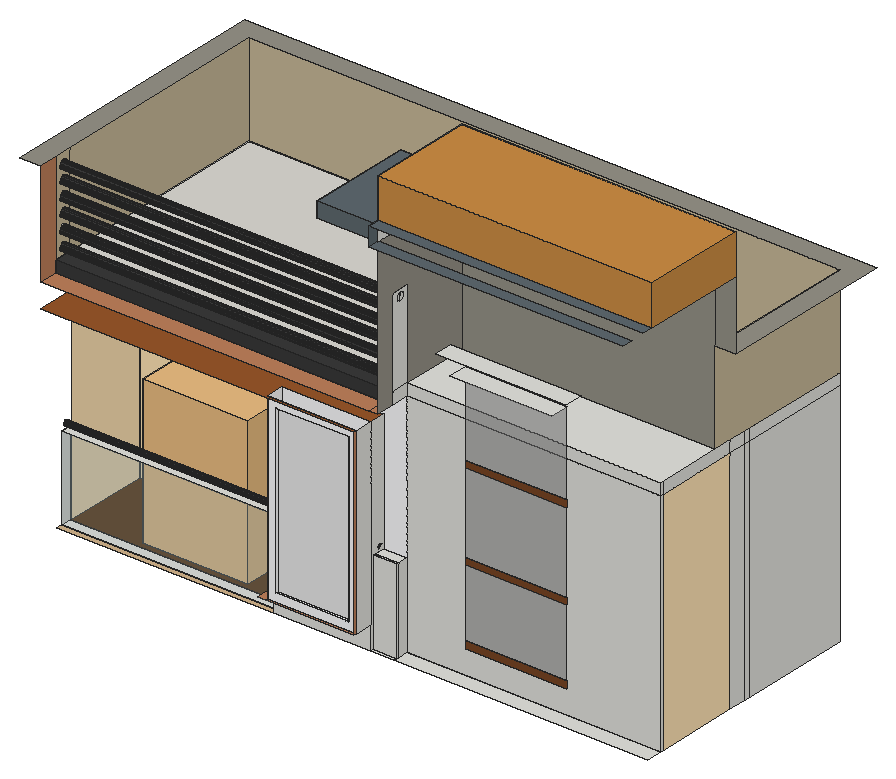
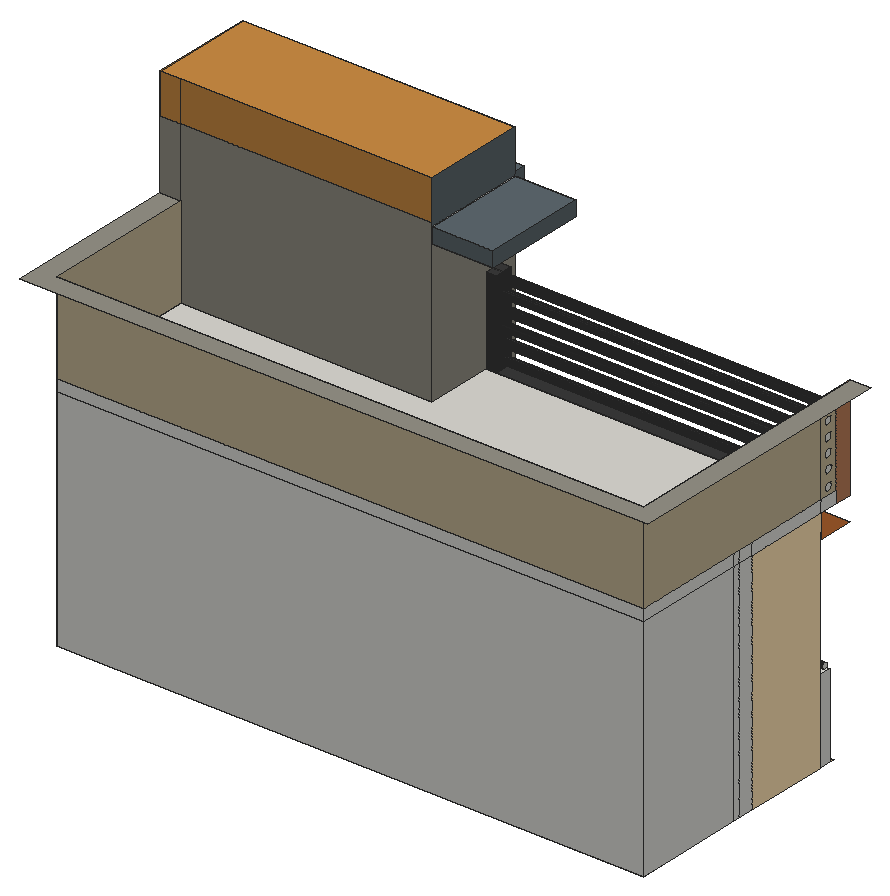
# SketchUp Ruby script. Lengths in inches.
U = 1.inch
M = Sketchup.active_model
def pt(a) = Geom::Point3d.new(a.map { |v| v * U })
def face(e, loops, mat)
  f = e.add_face(loops[0].map { |a| pt(a) })
  loops[1..].each { |l| e.add_face(l.map { |a| pt(a) }).erase! }
  f.material = f.back_material = mat if mat
  f
end
# faces: each face lists its corners as indices into pts; further lists are holes
def faces(e, pts, list, mat = nil) = list.each { |f| face(e, (f[0].is_a?(Array) ? f : [f]).map { |l| l.map { |i| pts[i] } }, mat) }
# xy, xz, yz: faces in a plane at the given z, y or x. An outline is a flat list of corners, or four numbers for a rectangle; further outlines are holes
def ring(l) = l.size == 4 ? [[l[0], l[1]], [l[2], l[1]], [l[2], l[3]], [l[0], l[3]]] : l.each_slice(2).to_a
def flat(e, list, mat, &to3) = list.each { |f| face(e, (f[0].is_a?(Array) ? f : [f]).map { |l| ring(l).map { |u, v| to3.(u, v) } }, mat) }
def xy(e, z, list, mat = nil) = flat(e, list, mat) { |x, y| [x, y, z] }
def xz(e, y, list, mat = nil) = flat(e, list, mat) { |x, z| [x, y, z] }
def yz(e, x, list, mat = nil) = flat(e, list, mat) { |y, z| [x, y, z] }
def lines(e, pts, list) = list.each { |a, b| e.add_line(pt(pts[a]), pt(pts[b])) }
# prism: a flat outline (further loops are holes) pulled along v
def prism(e, loops, v, mat = nil)
  f = face(e, loops, mat); d = Geom::Vector3d.new(v.map { |x| x * U })
  f.pushpull(f.normal.samedirection?(d) ? d.length : -d.length)
end
def box(e, o, s, mat = nil) = prism(e, [[o, [o[0] + s[0], o[1], o[2]], [o[0] + s[0], o[1] + s[1], o[2]], [o[0], o[1] + s[1], o[2]]]], [0, 0, s[2]], mat)
def at(x, y, z, deg = 0) = Geom::Transformation.translation(pt([x, y, z])) * Geom::Transformation.rotation(ORIGIN, Z_AXIS, deg.degrees)
def axes(o, x, y, z) = Geom::Transformation.new([*x, 0, *y, 0, *z, 0, *pt(o).to_a, 1])
def part(name) = M.definitions.add(name)
# library, detail: a bought-in or finely detailed component or shape, given as its bounding box
def library(name, o, s) = part(name).tap { |d| box(d.entities, o, s) }
def detail(e, o, s) = box(e.add_group.entities, o, s)
def put(e, d, t, mat = nil) = e.add_instance(d, t).tap { |i| i.material = mat if mat }
def group(e, t, mat = nil) = e.add_group.tap { |g| g.transformation = t; g.material = mat if mat }.entities
root = M.entities
M.materials.add("[0032_Moccasin]").color = [255, 228, 181]
M.materials.add("[0035_Tan]").color = [210, 180, 140]
M.materials.add("[Color M01]").color = [226, 226, 226]
M.materials.add("[Color M07]").color = [58, 58, 58]
M.materials.add("[Formica Graystone]").color = [149, 146, 135]
M.materials.add("[Formica Speckled Grey]").color = [94, 105, 111]
M.materials.add("[Leather Red Brown]").color = [76, 40, 8]
M.materials.add("[Quartz Light Brown]").color = [199, 184, 152]
M.materials.add("[Quartz Light Grey]").color = [251, 251, 252]
M.materials.add("[Sketchy Crosshatch Wavy]").color = [233, 233, 233]
M.materials.add("[Terrazzo Tile Light]").color = [219, 217, 210]
M.materials.add("[Translucent Glass Gray]").color = [128, 128, 128]
M.materials["[Translucent Glass Gray]"].alpha = 0.5
M.materials.add("[Translucent Glass Safety]").color = [204, 235, 244]
M.materials["[Translucent Glass Safety]"].alpha = 0.14
M.materials.add("[Wallpaper Stripe]").color = [204, 141, 68]
M.materials.add("[Wood Cherry Original]1").color = [152, 86, 42]
M.materials.add("[Wood Veneer 01]").color = [120, 70, 37]
M.materials.add("[Wood Veneer 02]").color = [190, 128, 91]
c1 = library("chau cay",[-24.34,-109.24,0],[56.46,62.58,79.69])
xy(root,394.8125,[[426.08,340.7,446.37,343.6],[446.37,340.7,663.13,354.64],[157.98,345.57,446.37,354.64],[157.98,428.92,663.13,448.59],[157.98,448.59,663.13,545.86]])
xy(root,394.8125,[[157.98,340.7,426.08,340.7,426.08,343.6,446.37,343.6,446.37,345.57,157.98,345.57]],"[0035_Tan]")
xy(root,394.8125,[[157.98,354.64,663.13,428.92]],"[Leather Red Brown]")
xy(root,414.6875,[[350.15,325.84,426.08,340.7]])
xy(root,414.6875,[[343.27,323.28,350.15,340.7],[350.15,323.28,426.08,325.84]],"[Wood Veneer 02]")
xy(root,421.41,[[356.87,325.84,419.36,328.53]],"[Quartz Light Grey]")
xy(root,467.1875,[[426.08,343.6,446.37,345.57],[157.98,345.57,426.08,354.64],[426.08,345.57,446.37,354.64]])
xy(root,563.42,[[356.87,325.84,419.36,328.53]],"[Quartz Light Grey]")
xy(root,570.15,[[157.98,323.28,157.98,354.64,426.08,354.64,426.08,340.7,350.15,340.7,350.15,325.84,426.08,325.84,426.08,323.28]],"[Wood Cherry Original]1")
xy(root,590.9375,[[157.98,338.96,446.37,354.64],[157.98,428.92,663.13,448.59],[157.98,448.59,663.13,545.86]])
xy(root,590.9375,[[157.98,354.64,663.13,428.92]],"[Wood Cherry Original]1")
xy(root,590.9375,[[157.98,323.28,438.32,338.96],[438.32,323.28,446.37,338.96]],"[Wood Veneer 02]")
xy(root,601.0625,[[446.37,354.64,663.13,412.7]])
xy(root,601.0625,[[157.98,338.96,437.35,354.64]],"[Color M07]")
xy(root,601.0625,[[157.98,354.64,446.37,354.64,446.37,412.7,663.13,412.7,663.13,545.86,157.98,545.86]],"[Terrazzo Tile Light]")
xy(root,653.58,[[521.21,307.03,607.83,323.28]])
xy(root,665.95,[[508.84,307.03,620.21,323.28]])
xy(root,676.1875,[[437.35,338.96,446.37,354.64]],"[Color M07]")
xy(root,680.125,[[140.56,323.28,157.98,323.28,157.98,545.86,663.13,545.86,663.13,412.7,680.56,412.7,680.56,563.28,140.56,563.28]],"[Formica Graystone]")
xy(root,723.1,[[394.12,323.28,446.37,412.7]],"[Color M01]")
xy(root,723.61,[[446.37,313.84,663.13,323.28]],"[Formica Speckled Grey]")
xy(root,736.05,[[394.12,323.28,446.37,412.7]],"[Formica Speckled Grey]")
xy(root,739.5,[[446.37,313.84,680.56,323.28]],"[Formica Speckled Grey]")
xy(root,773.8125,[[446.37,323.28,680.56,412.7]],"[Wallpaper Stripe]")
xz(root,323.28,[[394.12,723.1,446.37,736.05]],"[Formica Speckled Grey]")
xz(root,323.28,[[521.21,443.41,607.83,501.56],[521.21,507.35,607.83,576.06],[521.21,581.85,607.83,653.58]],"[Translucent Glass Gray]")
xz(root,323.28,[[446.37,739.5,680.56,773.8125]],"[Wallpaper Stripe]")
xz(root,323.28,[[521.21,437.62,607.83,443.41],[521.21,501.56,607.83,507.35],[521.21,576.06,607.83,581.85]],"[Wood Veneer 01]")
xz(root,325.84,[[[350.15,414.6875,426.08,570.15],[356.87,421.41,419.36,563.42]]],"[Quartz Light Grey]")
xz(root,328.53,[[356.87,421.41,419.36,563.42]],"[Sketchy Crosshatch Wavy]")
xz(root,338.96,[[157.98,590.9375,446.37,590.9375,446.37,676.1875,437.35,676.1875,437.35,601.0625,157.98,601.0625]],"[Color M07]")
xz(root,340.7,[[343.27,394.8125,426.08,414.6875]])
xz(root,340.7,[[350.15,414.6875,426.08,570.15]],"[Quartz Light Grey]")
xz(root,343.6,[[426.08,394.8125,446.37,467.1875]])
xz(root,345.57,[[157.98,394.8125,446.37,467.1875]],"[Translucent Glass Safety]")
xz(root,354.64,[[446.37,394.8125,663.13,590.9375],[157.98,590.9375,446.37,601.0625],[446.37,590.9375,663.13,601.0625]])
xz(root,354.64,[[437.35,601.0625,446.37,676.1875]],"[Color M07]")
xz(root,354.64,[[426.08,467.1875,426.08,570.15,157.98,570.15,157.98,590.9375,446.37,590.9375,446.37,467.1875]],"[Quartz Light Grey]")
xz(root,354.64,[[157.98,394.8125,446.37,467.1875]],"[Translucent Glass Safety]")
xz(root,412.7,[[446.37,601.0625,663.13,739.5],[663.13,680.125,680.56,739.5]],"[Formica Graystone]")
xz(root,412.7,[[394.12,723.1,446.37,736.05]],"[Formica Speckled Grey]")
xz(root,412.7,[[446.37,739.5,663.13,773.8125],[663.13,739.5,680.56,773.8125]],"[Wallpaper Stripe]")
xz(root,428.92,[[157.98,394.8125,663.13,590.9375]],"[0032_Moccasin]")
xz(root,448.59,[[157.98,394.8125,663.13,590.9375]])
xz(root,545.86,[[157.98,394.8125,663.13,590.9375],[157.98,590.9375,663.13,601.0625]])
xz(root,545.86,[[157.98,601.0625,663.13,680.125]],"[Quartz Light Brown]")
yz(root,157.98,[[345.57,394.8125,354.64,467.1875],[428.92,394.8125,443.28,590.9375],[443.28,394.8125,448.59,590.9375],[448.59,394.8125,545.86,590.9375],[350.17,469.16,349.6,469.23,349.07,469.45,348.62,469.8,348.27,470.25,348.05,470.78,347.98,471.34,348.05,471.91,348.27,472.4375,348.62,472.89,349.07,473.24,349.6,473.46,350.17,473.53,350.73,473.46,351.26,473.24,351.71,472.89,352.06,472.4375,352.28,471.91,352.35,471.34,352.28,470.78,352.06,470.25,351.71,469.8,351.26,469.45,350.73,469.23],
  [338.96,590.9375,354.64,601.0625],[354.64,590.9375,428.92,601.0625],[428.92,590.9375,443.28,601.0625],[443.28,590.9375,448.59,601.0625],[448.59,590.9375,545.86,601.0625],
  [346.73,604.61,345.84,604.73,345.01,605.07,344.3,605.62,343.76,606.33,343.41,607.16,343.3,608.05,343.41,608.94,343.76,609.77,344.3,610.48,345.01,611.03,345.84,611.37,346.73,611.49,347.625,611.37,348.45,611.03,349.16,610.48,349.71,609.77,350.05,608.94,350.17,608.05,350.05,607.16,349.71,606.33,349.16,605.62,348.45,605.07,347.625,604.73],[346.73,618.11,345.84,618.23,345.01,618.57,344.3,619.12,343.76,619.83,343.41,620.66,343.3,621.55,343.41,622.44,343.76,623.27,344.3,623.98,345.01,624.53,345.84,624.87,346.73,624.99,347.625,624.87,348.45,624.53,349.16,623.98,349.71,623.27,350.05,622.44,350.17,621.55,350.05,620.66,349.71,619.83,349.16,619.12,348.45,618.57,347.625,618.23],[347.05,630.54,346.16,630.65,345.33,631,344.62,631.54,344.08,632.26,343.73,633.08,343.62,633.97,343.73,634.86,344.08,635.69,344.62,636.4,345.33,636.95,346.16,637.29,347.05,637.41,347.94,637.29,348.77,636.95,349.48,636.4,350.03,635.69,350.37,634.86,350.49,633.97,350.37,633.08,350.03,632.26,349.48,631.54,348.77,631,347.94,630.65],[347.05,643.1,346.16,643.22,345.33,643.56,344.62,644.11,344.08,644.82,343.73,645.65,343.62,646.54,343.73,647.43,344.08,648.26,344.62,648.97,345.33,649.51,346.16,649.86,347.05,649.97,347.94,649.86,348.77,649.51,349.48,648.97,350.03,648.26,350.37,647.43,350.49,646.54,350.37,645.65,350.03,644.82,349.48,644.11,348.77,643.56,347.94,643.22],[347.05,655.79,346.16,655.9,345.33,656.25,344.62,656.79,344.08,657.51,343.73,658.33,343.62,659.22,343.73,660.11,344.08,660.94,344.62,661.65,345.33,662.2,346.16,662.54,347.05,662.66,347.94,662.54,348.77,662.2,349.48,661.65,350.03,660.94,350.37,660.11,350.49,659.22,350.37,658.33,350.03,657.51,349.48,656.79,348.77,656.25,347.94,655.9],
  [346.73,667.55,345.84,667.67,345.01,668.01,344.3,668.56,343.76,669.27,343.41,670.1,343.3,670.99,343.41,671.88,343.76,672.71,344.3,673.42,345.01,673.96,345.84,674.31,346.73,674.43,347.625,674.31,348.45,673.96,349.16,673.42,349.71,672.71,350.05,671.88,350.17,670.99,350.05,670.1,349.71,669.27,349.16,668.56,348.45,668.01,347.625,667.67]])
yz(root,157.98,[[356.33,394.8125,428.92,394.8125,428.92,590.9375,354.64,590.9375,354.64,576.33,356.33,576.33]],"[0032_Moccasin]")
yz(root,157.98,[[[338.96,601.0625,354.64,680.125],[346.73,667.55,345.84,667.67,345.01,668.01,344.3,668.56,343.76,669.27,343.41,670.1,343.3,670.99,343.41,671.88,343.76,672.71,344.3,673.42,345.01,673.96,345.84,674.31,346.73,674.43,347.625,674.31,348.45,673.96,349.16,673.42,349.71,672.71,350.05,671.88,350.17,670.99,350.05,670.1,349.71,669.27,349.16,668.56,348.45,668.01,347.625,667.67],[346.73,618.11,345.84,618.23,345.01,618.57,344.3,619.12,343.76,619.83,343.41,620.66,343.3,621.55,343.41,622.44,343.76,623.27,344.3,623.98,345.01,624.53,345.84,624.87,346.73,624.99,347.625,624.87,348.45,624.53,349.16,623.98,349.71,623.27,350.05,622.44,350.17,621.55,350.05,620.66,349.71,619.83,349.16,619.12,348.45,618.57,347.625,618.23],[347.05,655.79,346.16,655.9,345.33,656.25,344.62,656.79,344.08,657.51,343.73,658.33,343.62,659.22,343.73,660.11,344.08,660.94,344.62,661.65,345.33,662.2,346.16,662.54,347.05,662.66,347.94,662.54,348.77,662.2,349.48,661.65,350.03,660.94,350.37,660.11,350.49,659.22,350.37,658.33,350.03,657.51,349.48,656.79,348.77,656.25,347.94,655.9],[347.05,630.54,346.16,630.65,345.33,631,344.62,631.54,344.08,632.26,343.73,633.08,343.62,633.97,343.73,634.86,344.08,635.69,344.62,636.4,345.33,636.95,346.16,637.29,347.05,637.41,347.94,637.29,348.77,636.95,349.48,636.4,350.03,635.69,350.37,634.86,350.49,633.97,350.37,633.08,350.03,632.26,349.48,631.54,348.77,631,347.94,630.65],[347.05,643.1,346.16,643.22,345.33,643.56,344.62,644.11,344.08,644.82,343.73,645.65,343.62,646.54,343.73,647.43,344.08,648.26,344.62,648.97,345.33,649.51,346.16,649.86,347.05,649.97,347.94,649.86,348.77,649.51,349.48,648.97,350.03,648.26,350.37,647.43,350.49,646.54,350.37,645.65,350.03,644.82,349.48,644.11,348.77,643.56,347.94,643.22],[346.73,604.61,345.84,604.73,345.01,605.07,344.3,605.62,343.76,606.33,343.41,607.16,343.3,608.05,343.41,608.94,343.76,609.77,344.3,610.48,345.01,611.03,345.84,611.37,346.73,611.49,347.625,611.37,348.45,611.03,349.16,610.48,349.71,609.77,350.05,608.94,350.17,608.05,350.05,607.16,349.71,606.33,349.16,605.62,348.45,605.07,347.625,604.73]],[354.64,601.0625,545.86,680.125]],"[Quartz Light Brown]")
yz(root,157.98,[[323.28,590.9375,338.96,680.125]],"[Wood Veneer 02]")
yz(root,350.15,[[325.84,414.6875,340.7,570.15]],"[Quartz Light Grey]")
yz(root,356.87,[[325.84,421.41,328.53,563.42]],"[Quartz Light Grey]")
yz(root,394.12,[[323.28,723.1,412.7,736.05]],"[Formica Speckled Grey]")
yz(root,419.36,[[325.84,421.41,328.53,563.42]])
yz(root,426.08,[[[340.7,394.8125,340.7,570.15,354.64,570.15,354.64,467.1875,343.6,467.1875,343.6,394.8125],[350.17,469.16,350.73,469.23,351.26,469.45,351.71,469.8,352.06,470.25,352.28,470.78,352.35,471.34,352.28,471.91,352.06,472.4375,351.71,472.89,351.26,473.24,350.73,473.46,350.17,473.53,349.6,473.46,349.07,473.24,348.62,472.89,348.27,472.4375,348.05,471.91,347.98,471.34,348.05,470.78,348.27,470.25,348.62,469.8,349.07,469.45,349.6,469.23]],[325.84,414.6875,340.7,570.15]])
yz(root,426.08,[[323.28,414.6875,325.84,570.15]],"[Wood Veneer 02]")
yz(root,437.35,[[[338.96,601.0625,354.64,676.1875],[347.05,655.79,347.94,655.9,348.77,656.25,349.48,656.79,350.03,657.51,350.37,658.33,350.49,659.22,350.37,660.11,350.03,660.94,349.48,661.65,348.77,662.2,347.94,662.54,347.05,662.66,346.16,662.54,345.33,662.2,344.62,661.65,344.08,660.94,343.73,660.11,343.62,659.22,343.73,658.33,344.08,657.51,344.62,656.79,345.33,656.25,346.16,655.9],[347.05,643.1,347.94,643.22,348.77,643.56,349.48,644.11,350.03,644.82,350.37,645.65,350.49,646.54,350.37,647.43,350.03,648.26,349.48,648.97,348.77,649.51,347.94,649.86,347.05,649.97,346.16,649.86,345.33,649.51,344.62,648.97,344.08,648.26,343.73,647.43,343.62,646.54,343.73,645.65,344.08,644.82,344.62,644.11,345.33,643.56,346.16,643.22],[346.73,604.61,347.625,604.73,348.45,605.07,349.16,605.62,349.71,606.33,350.05,607.16,350.17,608.05,350.05,608.94,349.71,609.77,349.16,610.48,348.45,611.03,347.625,611.37,346.73,611.49,345.84,611.37,345.01,611.03,344.3,610.48,343.76,609.77,343.41,608.94,343.3,608.05,343.41,607.16,343.76,606.33,344.3,605.62,345.01,605.07,345.84,604.73],[346.73,618.11,347.625,618.23,348.45,618.57,349.16,619.12,349.71,619.83,350.05,620.66,350.17,621.55,350.05,622.44,349.71,623.27,349.16,623.98,348.45,624.53,347.625,624.87,346.73,624.99,345.84,624.87,345.01,624.53,344.3,623.98,343.76,623.27,343.41,622.44,343.3,621.55,343.41,620.66,343.76,619.83,344.3,619.12,345.01,618.57,345.84,618.23],[347.05,630.54,347.94,630.65,348.77,631,349.48,631.54,350.03,632.26,350.37,633.08,350.49,633.97,350.37,634.86,350.03,635.69,349.48,636.4,348.77,636.95,347.94,637.29,347.05,637.41,346.16,637.29,345.33,636.95,344.62,636.4,344.08,635.69,343.73,634.86,343.62,633.97,343.73,633.08,344.08,632.26,344.62,631.54,345.33,631,346.16,630.65]]],"[Color M07]")
yz(root,446.37,[[343.6,394.8125,345.57,467.1875],[345.57,394.8125,354.64,467.1875],[338.96,590.9375,354.64,601.0625],[338.96,601.0625,354.64,601.0625,354.64,676.1875,346.83,676.1875,346.83,674.41,347.625,674.31,348.45,673.96,349.16,673.42,349.71,672.71,350.05,671.88,350.17,670.99,350.05,670.1,349.71,669.27,349.16,668.56,348.45,668.01,347.625,667.67,346.83,667.5625,346.73,667.55,346.64,667.5625,345.84,667.67,345.01,668.01,344.3,668.56,343.76,669.27,343.41,670.1,343.3,670.99,343.41,671.88,343.76,672.71,344.3,673.42,345.01,673.96,345.84,674.31,346.64,674.41,346.64,676.1875,338.96,676.1875],[[338.96,601.0625,354.64,676.1875],[346.73,667.55,346.83,667.5625,347.625,667.67,348.45,668.01,349.16,668.56,349.71,669.27,350.05,670.1,350.17,670.99,350.05,671.88,349.71,672.71,349.16,673.42,348.45,673.96,347.625,674.31,346.83,674.41,346.73,674.43,346.64,674.41,345.84,674.31,345.01,673.96,344.3,673.42,343.76,672.71,343.41,671.88,343.3,670.99,343.41,670.1,343.76,669.27,344.3,668.56,345.01,668.01,345.84,667.67,346.64,667.5625]],
  [346.73,667.55,346.83,667.5625,346.83,674.41,346.73,674.43,346.64,674.41,346.64,667.5625],[346.64,667.5625,346.64,674.41,345.84,674.31,345.01,673.96,344.3,673.42,343.76,672.71,343.41,671.88,343.3,670.99,343.41,670.1,343.76,669.27,344.3,668.56,345.01,668.01,345.84,667.67],[346.83,667.5625,347.625,667.67,348.45,668.01,349.16,668.56,349.71,669.27,350.05,670.1,350.17,670.99,350.05,671.88,349.71,672.71,349.16,673.42,348.45,673.96,347.625,674.31,346.83,674.41],[346.64,674.41,346.73,674.43,346.83,674.41,346.83,676.1875,346.64,676.1875],[323.28,723.1,412.7,736.05]])
yz(root,446.37,[[323.28,590.9375,323.28,723.1,412.7,723.1,412.7,601.0625,354.64,601.0625,354.64,676.1875,338.96,676.1875,338.96,590.9375]],"[Formica Graystone]")
yz(root,446.37,[[313.84,723.61,323.28,739.5],[323.28,736.05,412.7,773.8125]],"[Formica Speckled Grey]")
yz(root,663.13,[[354.64,394.8125,356.33,590.9375],[428.92,394.8125,443.28,590.9375],[443.28,394.8125,448.59,590.9375],[448.59,394.8125,545.86,590.9375],[354.64,590.9375,356.33,601.0625],
  [356.33,590.9375,428.92,601.0625],[428.92,590.9375,443.28,601.0625],[443.28,590.9375,448.59,601.0625],[448.59,590.9375,545.86,601.0625]])
yz(root,663.13,[[356.33,394.8125,428.92,590.9375]],"[0032_Moccasin]")
yz(root,663.13,[[412.7,601.0625,545.86,680.125]],"[Quartz Light Brown]")
yz(root,680.56,[[323.28,739.5,412.7,773.8125]],"[Wallpaper Stripe]")
p = [[157.98,349.07,469.45],[157.98,349.6,469.23],[426.08,349.6,469.23],[426.08,349.07,469.45],[157.98,350.17,469.16],[426.08,350.17,469.16],
  [157.98,350.73,469.23],[426.08,350.73,469.23],[157.98,351.26,469.45],[426.08,351.26,469.45],[157.98,348.62,469.8],[426.08,348.62,469.8],
  [157.98,351.71,469.8],[426.08,351.71,469.8],[157.98,348.27,470.25],[426.08,348.27,470.25],[157.98,352.06,470.25],[426.08,352.06,470.25],
  [157.98,348.05,470.78],[426.08,348.05,470.78],[157.98,352.28,470.78],[426.08,352.28,470.78],[157.98,347.98,471.34],[426.08,347.98,471.34],
  [157.98,352.35,471.34],[426.08,352.35,471.34],[157.98,348.05,471.91],[426.08,348.05,471.91],[157.98,352.28,471.91],[426.08,352.28,471.91],
  [157.98,348.27,472.4375],[426.08,348.27,472.4375],[157.98,352.06,472.4375],[426.08,352.06,472.4375],[157.98,348.62,472.89],[426.08,348.62,472.89],
  [157.98,351.71,472.89],[426.08,351.71,472.89],[157.98,349.07,473.24],[426.08,349.07,473.24],[157.98,351.26,473.24],[426.08,351.26,473.24],
  [157.98,349.6,473.46],[426.08,349.6,473.46],[157.98,350.73,473.46],[426.08,350.73,473.46],[157.98,350.17,473.53],[426.08,350.17,473.53],
  [157.98,345.84,604.73],[157.98,346.73,604.61],[437.35,346.73,604.61],[437.35,345.84,604.73],[157.98,347.625,604.73],[437.35,347.625,604.73],
  [157.98,345.01,605.07],[437.35,345.01,605.07],[157.98,348.45,605.07],[437.35,348.45,605.07],[157.98,344.3,605.62],[437.35,344.3,605.62],
  [157.98,349.16,605.62],[437.35,349.16,605.62],[157.98,343.76,606.33],[437.35,343.76,606.33],[157.98,349.71,606.33],[437.35,349.71,606.33],
  [157.98,343.41,607.16],[437.35,343.41,607.16],[157.98,350.05,607.16],[437.35,350.05,607.16],[157.98,343.3,608.05],[437.35,343.3,608.05],
  [157.98,350.17,608.05],[437.35,350.17,608.05],[157.98,343.41,608.94],[437.35,343.41,608.94],[157.98,350.05,608.94],[437.35,350.05,608.94],
  [157.98,343.76,609.77],[437.35,343.76,609.77],[157.98,349.71,609.77],[437.35,349.71,609.77],[157.98,344.3,610.48],[437.35,344.3,610.48],
  [157.98,349.16,610.48],[437.35,349.16,610.48],[157.98,345.01,611.03],[437.35,345.01,611.03],[157.98,348.45,611.03],[437.35,348.45,611.03],
  [157.98,345.84,611.37],[437.35,345.84,611.37],[157.98,347.625,611.37],[437.35,347.625,611.37],[157.98,346.73,611.49],[437.35,346.73,611.49],
  [157.98,345.84,618.23],[157.98,346.73,618.11],[437.35,346.73,618.11],[437.35,345.84,618.23],[157.98,347.625,618.23],[437.35,347.625,618.23],
  [157.98,345.01,618.57],[437.35,345.01,618.57],[157.98,348.45,618.57],[437.35,348.45,618.57],[157.98,344.3,619.12],[437.35,344.3,619.12],
  [157.98,349.16,619.12],[437.35,349.16,619.12],[157.98,343.76,619.83],[437.35,343.76,619.83],[157.98,349.71,619.83],[437.35,349.71,619.83],
  [157.98,343.41,620.66],[437.35,343.41,620.66],[157.98,350.05,620.66],[437.35,350.05,620.66],[157.98,343.3,621.55],[437.35,343.3,621.55],
  [157.98,350.17,621.55],[437.35,350.17,621.55],[157.98,343.41,622.44],[437.35,343.41,622.44],[157.98,350.05,622.44],[437.35,350.05,622.44],
  [157.98,343.76,623.27],[437.35,343.76,623.27],[157.98,349.71,623.27],[437.35,349.71,623.27],[157.98,344.3,623.98],[437.35,344.3,623.98],
  [157.98,349.16,623.98],[437.35,349.16,623.98],[157.98,345.01,624.53],[437.35,345.01,624.53],[157.98,348.45,624.53],[437.35,348.45,624.53],
  [157.98,345.84,624.87],[437.35,345.84,624.87],[157.98,347.625,624.87],[437.35,347.625,624.87],[157.98,346.73,624.99],[437.35,346.73,624.99],
  [157.98,346.16,630.65],[157.98,347.05,630.54],[437.35,347.05,630.54],[437.35,346.16,630.65],[157.98,347.94,630.65],[437.35,347.94,630.65],
  [157.98,345.33,631],[437.35,345.33,631],[157.98,348.77,631],[437.35,348.77,631],[157.98,344.62,631.54],[437.35,344.62,631.54],
  [157.98,349.48,631.54],[437.35,349.48,631.54],[157.98,344.08,632.26],[437.35,344.08,632.26],[157.98,350.03,632.26],[437.35,350.03,632.26],
  [157.98,343.73,633.08],[437.35,343.73,633.08],[157.98,350.37,633.08],[437.35,350.37,633.08],[157.98,343.62,633.97],[437.35,343.62,633.97],
  [157.98,350.49,633.97],[437.35,350.49,633.97],[157.98,343.73,634.86],[437.35,343.73,634.86],[157.98,350.37,634.86],[437.35,350.37,634.86],
  [157.98,344.08,635.69],[437.35,344.08,635.69],[157.98,350.03,635.69],[437.35,350.03,635.69],[157.98,344.62,636.4],[437.35,344.62,636.4],
  [157.98,349.48,636.4],[437.35,349.48,636.4],[157.98,345.33,636.95],[437.35,345.33,636.95],[157.98,348.77,636.95],[437.35,348.77,636.95],
  [157.98,346.16,637.29],[437.35,346.16,637.29],[157.98,347.94,637.29],[437.35,347.94,637.29],[157.98,347.05,637.41],[437.35,347.05,637.41],
  [157.98,346.16,643.22],[157.98,347.05,643.1],[437.35,347.05,643.1],[437.35,346.16,643.22],[157.98,347.94,643.22],[437.35,347.94,643.22],
  [157.98,345.33,643.56],[437.35,345.33,643.56],[157.98,348.77,643.56],[437.35,348.77,643.56],[157.98,344.62,644.11],[437.35,344.62,644.11],
  [157.98,349.48,644.11],[437.35,349.48,644.11],[157.98,344.08,644.82],[437.35,344.08,644.82],[157.98,350.03,644.82],[437.35,350.03,644.82],
  [157.98,343.73,645.65],[437.35,343.73,645.65],[157.98,350.37,645.65],[437.35,350.37,645.65],[157.98,343.62,646.54],[437.35,343.62,646.54],
  [157.98,350.49,646.54],[437.35,350.49,646.54],[157.98,343.73,647.43],[437.35,343.73,647.43],[157.98,350.37,647.43],[437.35,350.37,647.43],
  [157.98,344.08,648.26],[437.35,344.08,648.26],[157.98,350.03,648.26],[437.35,350.03,648.26],[157.98,344.62,648.97],[437.35,344.62,648.97],
  [157.98,349.48,648.97],[437.35,349.48,648.97],[157.98,345.33,649.51],[437.35,345.33,649.51],[157.98,348.77,649.51],[437.35,348.77,649.51],
  [157.98,346.16,649.86],[437.35,346.16,649.86],[157.98,347.94,649.86],[437.35,347.94,649.86],[157.98,347.05,649.97],[437.35,347.05,649.97],
  [157.98,346.16,655.9],[157.98,347.05,655.79],[437.35,347.05,655.79],[437.35,346.16,655.9],[157.98,347.94,655.9],[437.35,347.94,655.9],
  [157.98,345.33,656.25],[437.35,345.33,656.25],[157.98,348.77,656.25],[437.35,348.77,656.25],[157.98,344.62,656.79],[437.35,344.62,656.79],
  [157.98,349.48,656.79],[437.35,349.48,656.79],[157.98,344.08,657.51],[437.35,344.08,657.51],[157.98,350.03,657.51],[437.35,350.03,657.51],
  [157.98,343.73,658.33],[437.35,343.73,658.33],[157.98,350.37,658.33],[437.35,350.37,658.33],[157.98,343.62,659.22],[437.35,343.62,659.22],
  [157.98,350.49,659.22],[437.35,350.49,659.22],[157.98,343.73,660.11],[437.35,343.73,660.11],[157.98,350.37,660.11],[437.35,350.37,660.11],
  [157.98,344.08,660.94],[437.35,344.08,660.94],[157.98,350.03,660.94],[437.35,350.03,660.94],[157.98,344.62,661.65],[437.35,344.62,661.65],
  [157.98,349.48,661.65],[437.35,349.48,661.65],[157.98,345.33,662.2],[437.35,345.33,662.2],[157.98,348.77,662.2],[437.35,348.77,662.2],
  [157.98,346.16,662.54],[437.35,346.16,662.54],[157.98,347.94,662.54],[437.35,347.94,662.54],[157.98,347.05,662.66],[437.35,347.05,662.66],
  [157.98,345.84,667.67],[157.98,346.73,667.55],[446.37,346.73,667.55],[446.37,346.64,667.5625],[446.37,345.84,667.67],[157.98,347.625,667.67],
  [446.37,347.625,667.67],[446.37,346.83,667.5625],[157.98,345.01,668.01],[446.37,345.01,668.01],[157.98,348.45,668.01],[446.37,348.45,668.01],
  [157.98,344.3,668.56],[446.37,344.3,668.56],[157.98,349.16,668.56],[446.37,349.16,668.56],[157.98,343.76,669.27],[446.37,343.76,669.27],
  [157.98,349.71,669.27],[446.37,349.71,669.27],[157.98,343.41,670.1],[446.37,343.41,670.1],[157.98,350.05,670.1],[446.37,350.05,670.1],
  [157.98,343.3,670.99],[446.37,343.3,670.99],[157.98,350.17,670.99],[446.37,350.17,670.99],[157.98,343.41,671.88],[446.37,343.41,671.88],
  [157.98,350.05,671.88],[446.37,350.05,671.88],[157.98,343.76,672.71],[446.37,343.76,672.71],[157.98,349.71,672.71],[446.37,349.71,672.71],
  [157.98,344.3,673.42],[446.37,344.3,673.42],[157.98,349.16,673.42],[446.37,349.16,673.42],[157.98,345.01,673.96],[446.37,345.01,673.96],
  [157.98,348.45,673.96],[446.37,348.45,673.96],[157.98,345.84,674.31],[446.37,345.84,674.31],[157.98,347.625,674.31],[446.37,347.625,674.31],
  [157.98,346.73,674.43],[446.37,346.64,674.41],[446.37,346.73,674.43],[446.37,346.83,674.41]]
faces(root,p,[[0,1,2,3],[1,4,5,2],[4,6,7,5],[6,8,9,7],[10,0,3,11],[8,12,13,9],[14,10,11,15],[12,16,17,13],
  [18,14,15,19],[16,20,21,17],[22,18,19,23],[20,24,25,21],[26,22,23,27],[24,28,29,25],[30,26,27,31],[28,32,33,29],
  [34,30,31,35],[32,36,37,33],[38,34,35,39],[36,40,41,37],[42,38,39,43],[40,44,45,41],[46,42,43,47],[44,46,47,45],
  [48,49,50,51],[49,52,53,50],[54,48,51,55],[52,56,57,53],[58,54,55,59],[56,60,61,57],[62,58,59,63],[60,64,65,61],
  [66,62,63,67],[64,68,69,65],[70,66,67,71],[68,72,73,69],[74,70,71,75],[72,76,77,73],[78,74,75,79],[76,80,81,77],
  [82,78,79,83],[80,84,85,81],[86,82,83,87],[84,88,89,85],[90,86,87,91],[88,92,93,89],[94,90,91,95],[92,94,95,93],
  [96,97,98,99],[97,100,101,98],[102,96,99,103],[100,104,105,101],[106,102,103,107],[104,108,109,105],[110,106,107,111],[108,112,113,109],
  [114,110,111,115],[112,116,117,113],[118,114,115,119],[116,120,121,117],[122,118,119,123],[120,124,125,121],[126,122,123,127],[124,128,129,125],
  [130,126,127,131],[128,132,133,129],[134,130,131,135],[132,136,137,133],[138,134,135,139],[136,140,141,137],[142,138,139,143],[140,142,143,141],
  [144,145,146,147],[145,148,149,146],[150,144,147,151],[148,152,153,149],[154,150,151,155],[152,156,157,153],[158,154,155,159],[156,160,161,157],
  [162,158,159,163],[160,164,165,161],[166,162,163,167],[164,168,169,165],[170,166,167,171],[168,172,173,169],[174,170,171,175],[172,176,177,173],
  [178,174,175,179],[176,180,181,177],[182,178,179,183],[180,184,185,181],[186,182,183,187],[184,188,189,185],[190,186,187,191],[188,190,191,189],
  [192,193,194,195],[193,196,197,194],[198,192,195,199],[196,200,201,197],[202,198,199,203],[200,204,205,201],[206,202,203,207],[204,208,209,205],
  [210,206,207,211],[208,212,213,209],[214,210,211,215],[212,216,217,213],[218,214,215,219],[216,220,221,217],[222,218,219,223],[220,224,225,221],
  [226,222,223,227],[224,228,229,225],[230,226,227,231],[228,232,233,229],[234,230,231,235],[232,236,237,233],[238,234,235,239],[236,238,239,237],
  [240,241,242,243],[241,244,245,242],[246,240,243,247],[244,248,249,245],[250,246,247,251],[248,252,253,249],[254,250,251,255],[252,256,257,253],
  [258,254,255,259],[256,260,261,257],[262,258,259,263],[260,264,265,261],[266,262,263,267],[264,268,269,265],[270,266,267,271],[268,272,273,269],
  [274,270,271,275],[272,276,277,273],[278,274,275,279],[276,280,281,277],[282,278,279,283],[280,284,285,281],[286,282,283,287],[284,286,287,285],
  [288,289,290,291,292],[289,293,294,295,290],[296,288,292,297],[293,298,299,294],[300,296,297,301],[298,302,303,299],[304,300,301,305],[302,306,307,303],
  [308,304,305,309],[306,310,311,307],[312,308,309,313],[310,314,315,311],[316,312,313,317],[314,318,319,315],[320,316,317,321],[318,322,323,319],
  [324,320,321,325],[322,326,327,323],[328,324,325,329],[326,330,331,327],[332,328,329,333],[330,334,335,331],[336,332,333,337,338],[334,336,338,339,335]],"[Color M07]")
put(root,c1,axes([254.61,480.31,395.5],[1.596,0,0],[0,1.10136,0],[0,0,1.57183]))
